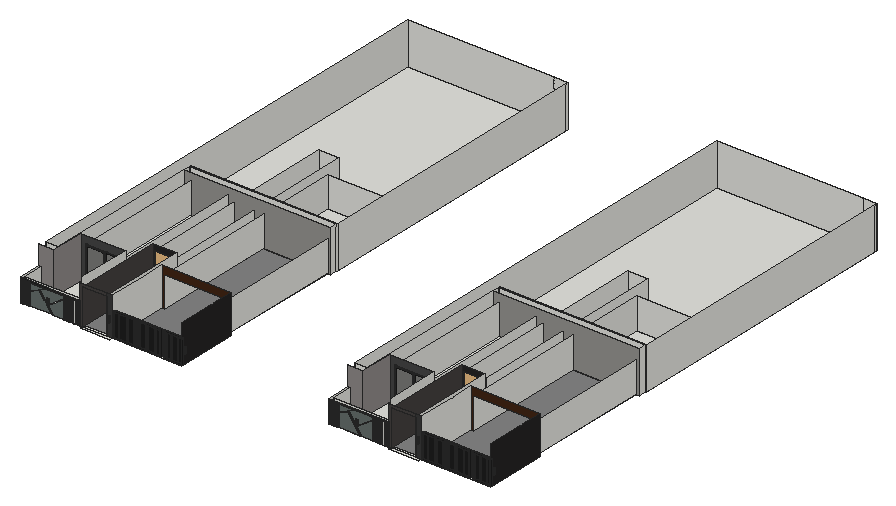
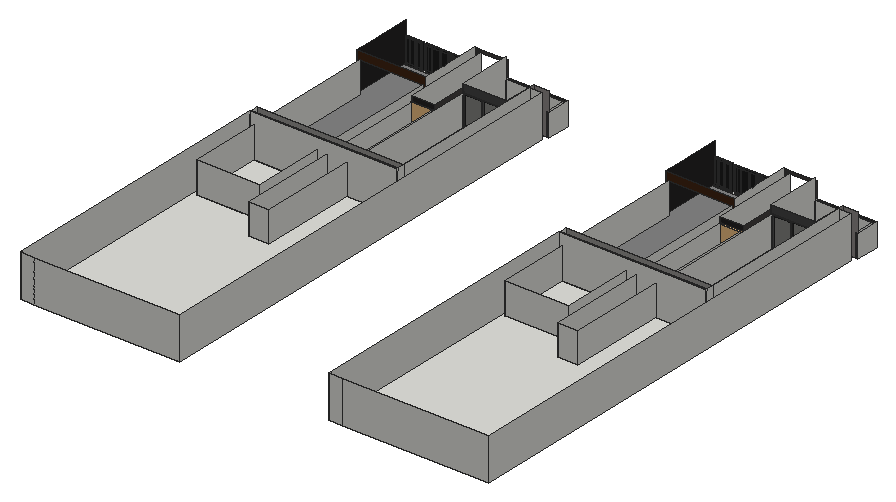
# SketchUp Ruby script. Lengths in inches.
U = 1.inch
M = Sketchup.active_model
def pt(a) = Geom::Point3d.new(a.map { |v| v * U })
def face(e, loops, mat)
  f = e.add_face(loops[0].map { |a| pt(a) })
  loops[1..].each { |l| e.add_face(l.map { |a| pt(a) }).erase! }
  f.material = f.back_material = mat if mat
  f
end
# faces: each face lists its corners as indices into pts; further lists are holes
def faces(e, pts, list, mat = nil) = list.each { |f| face(e, (f[0].is_a?(Array) ? f : [f]).map { |l| l.map { |i| pts[i] } }, mat) }
# xy, xz, yz: faces in a plane at the given z, y or x. An outline is a flat list of corners, or four numbers for a rectangle; further outlines are holes
def ring(l) = l.size == 4 ? [[l[0], l[1]], [l[2], l[1]], [l[2], l[3]], [l[0], l[3]]] : l.each_slice(2).to_a
def flat(e, list, mat, &to3) = list.each { |f| face(e, (f[0].is_a?(Array) ? f : [f]).map { |l| ring(l).map { |u, v| to3.(u, v) } }, mat) }
def xy(e, z, list, mat = nil) = flat(e, list, mat) { |x, y| [x, y, z] }
def xz(e, y, list, mat = nil) = flat(e, list, mat) { |x, z| [x, y, z] }
def yz(e, x, list, mat = nil) = flat(e, list, mat) { |y, z| [x, y, z] }
def lines(e, pts, list) = list.each { |a, b| e.add_line(pt(pts[a]), pt(pts[b])) }
# prism: a flat outline (further loops are holes) pulled along v
def prism(e, loops, v, mat = nil)
  f = face(e, loops, mat); d = Geom::Vector3d.new(v.map { |x| x * U })
  f.pushpull(f.normal.samedirection?(d) ? d.length : -d.length)
end
def box(e, o, s, mat = nil) = prism(e, [[o, [o[0] + s[0], o[1], o[2]], [o[0] + s[0], o[1] + s[1], o[2]], [o[0], o[1] + s[1], o[2]]]], [0, 0, s[2]], mat)
def at(x, y, z, deg = 0) = Geom::Transformation.translation(pt([x, y, z])) * Geom::Transformation.rotation(ORIGIN, Z_AXIS, deg.degrees)
def axes(o, x, y, z) = Geom::Transformation.new([*x, 0, *y, 0, *z, 0, *pt(o).to_a, 1])
def part(name) = M.definitions.add(name)
# library, detail: a bought-in or finely detailed component or shape, given as its bounding box
def library(name, o, s) = part(name).tap { |d| box(d.entities, o, s) }
def detail(e, o, s) = box(e.add_group.entities, o, s)
def put(e, d, t, mat = nil) = e.add_instance(d, t).tap { |i| i.material = mat if mat }
def group(e, t, mat = nil) = e.add_group.tap { |g| g.transformation = t; g.material = mat if mat }.entities
root = M.entities
M.materials.add("Glass_Tinted_Gray").color = [0, 0, 0]
M.materials["Glass_Tinted_Gray"].alpha = 0.125
M.materials.add("[0135_DarkGray]").color = [81, 81, 81]
M.materials.add("[Color M07]").color = [58, 58, 58]
M.materials.add("[Color M08]").color = [30, 30, 30]
M.materials.add("[Granite Dark Gray]").color = [38, 37, 37]
M.materials.add("[Granite Dark Gray]1").color = [69, 68, 68]
M.materials.add("[Granite Light Gray]").color = [149, 148, 144]
M.materials.add("[Granite Tile]1").color = [68, 65, 63]
M.materials.add("[Mirror 02]").color = [229, 229, 229]
M.materials.add("[Slate]").color = [102, 110, 108]
M.materials.add("[Stone Marble]").color = [143, 138, 136]
M.materials.add("[Terrazzo Light Blue]").color = [196, 214, 227]
M.materials.add("[Tile Grey]").color = [132, 132, 132]
M.materials.add("[Wood Veneer 01]").color = [66, 38, 20]
c1 = part("Group\#7")
xy(c1.entities,0,[[6,0,4.45,0.2,3,0.8,1.76,1.76,0.8,3,0.2,4.45,0,6,0.2,7.55,0.8,9,1.76,10.24,3,11.2,4.45,11.8,6,12,7.55,11.8,9,11.2,10.24,10.24,11.2,9,11.8,7.55,12,6,11.8,4.45,11.2,3,10.24,1.76,9,0.8,7.55,0.2]])
xy(c1.entities,37,[[6,0,7.55,0.2,9,0.8,10.24,1.76,11.2,3,11.8,4.45,12,6,11.8,7.55,11.2,9,10.24,10.24,9,11.2,7.55,11.8,6,12,4.45,11.8,3,11.2,1.76,10.24,0.8,9,0.2,7.55,0,6,0.2,4.45,0.8,3,1.76,1.76,3,0.8,4.45,0.2]],"[Granite Tile]1")
p = [[4.45,0.2,0],[6,0,0],[6,0,37],[4.45,0.2,37],[7.55,0.2,0],[7.55,0.2,37],
  [3,0.8,0],[3,0.8,37],[9,0.8,0],[9,0.8,37],[1.76,1.76,0],[1.76,1.76,37],
  [10.24,1.76,0],[10.24,1.76,37],[0.8,3,0],[0.8,3,37],[11.2,3,0],[11.2,3,37],
  [0.2,4.45,0],[0.2,4.45,37],[11.8,4.45,0],[11.8,4.45,37],[0,6,0],[0,6,37],
  [12,6,0],[12,6,37],[0.2,7.55,0],[0.2,7.55,37],[11.8,7.55,0],[11.8,7.55,37],
  [0.8,9,0],[0.8,9,37],[11.2,9,0],[11.2,9,37],[1.76,10.24,0],[1.76,10.24,37],
  [10.24,10.24,0],[10.24,10.24,37],[3,11.2,0],[3,11.2,37],[9,11.2,0],[9,11.2,37],
  [4.45,11.8,0],[4.45,11.8,37],[7.55,11.8,0],[7.55,11.8,37],[6,12,0],[6,12,37]]
faces(c1.entities,p,[[0,1,2,3],[1,4,5,2],[6,0,3,7],[4,8,9,5],[10,6,7,11],[8,12,13,9],[14,10,11,15],[12,16,17,13],
  [18,14,15,19],[16,20,21,17],[22,18,19,23],[20,24,25,21],[26,22,23,27],[24,28,29,25],[30,26,27,31],[28,32,33,29],
  [34,30,31,35],[32,36,37,33],[38,34,35,39],[36,40,41,37],[42,38,39,43],[40,44,45,41],[46,42,43,47],[44,46,47,45]],"[Granite Tile]1")
c2 = part("PENTEK_RP Fineline 50S_Sliding_DoorCase_E1")
box(c2.entities,[0,0,0],[1.51,3.66,99.27],"[0135_DarkGray]")
c3 = part("PENTEK_RP Fineline 50S_SlidingDooe_Case_E2")
box(c3.entities,[0,0,0],[96.25,3.66,1.51],"[0135_DarkGray]")
c4 = part("pentek_RP Fineline 50S_SlidingDoor_Case")
put(c4.entities,c2,at(97.76,0,0))
put(c4.entities,c3,at(1.51,0,0))
put(c4.entities,c2,at(0,0,0))
put(c4.entities,c3,at(1.51,0,97.76))
c5 = part("PENTEK_RP Fineline 50S_SlidingDoor_GlazingBead_2")
box(c5.entities,[0,0,0],[0.56,0.59,94.39],"[0135_DarkGray]")
c6 = part("PENTEK_RP Fineline 50S_SlidingDoor_Glass")
box(c6.entities,[0,0,0],[46.58,0.16,94.39],"Glass_Tinted_Gray")
c7 = part("PENTEK_RP Fineline 50S_SlidingDoor_GlazingBead")
box(c7.entities,[0,0,0],[45.47,0.59,0.56],"[0135_DarkGray]")
c8 = part("PENTEK_RP Fineline 50S_SlidingDoor_Leaf_E1")
xy(c8.entities,0,[[0,0,0.93,1.97],[0.93,1.57,1.49,1.97]],"[0135_DarkGray]")
xy(c8.entities,96.25,[[0,0,0.93,0,0.93,1.57,1.49,1.57,1.49,1.97,0,1.97]],"[0135_DarkGray]")
xz(c8.entities,0,[[0,0,0.93,96.25]],"[0135_DarkGray]")
xz(c8.entities,1.57,[[0.93,0,1.49,95.32],[0.93,95.32,1.49,96.25]],"[0135_DarkGray]")
xz(c8.entities,1.97,[[0,0,1.49,96.25]],"[0135_DarkGray]")
yz(c8.entities,0,[[0,0,1.97,96.25]],"[0135_DarkGray]")
yz(c8.entities,0.93,[[0,0,1.57,0.93],[0,0.93,1.57,95.32],[0,95.32,1.57,96.25]],"[0135_DarkGray]")
yz(c8.entities,1.49,[[1.57,0,1.97,95.32],[1.57,95.32,1.97,96.25]],"[0135_DarkGray]")
c9 = part("PENTEK_RP Fineline 50S_SlidingDoor_Leaf_E2")
xy(c9.entities,0,[[0,0,0,1.57,0.56,1.57,0.56,1.97,46.02,1.97,46.02,1.57,46.58,1.57,46.58,0]],"[0135_DarkGray]")
xy(c9.entities,0.93,[[0,0,46.58,1.57]],"[0135_DarkGray]")
xy(c9.entities,1.49,[[0.56,1.57,46.02,1.97]],"[0135_DarkGray]")
xz(c9.entities,0,[[0,0,46.58,0.93]],"[0135_DarkGray]")
xz(c9.entities,1.57,[[0,0,0.56,0.93],[46.02,0,46.58,0.93],[0.56,0.93,46.02,1.49]],"[0135_DarkGray]")
xz(c9.entities,1.97,[[0.56,0,46.02,1.49]],"[0135_DarkGray]")
yz(c9.entities,0,[[0,0,1.57,0.93]],"[0135_DarkGray]")
yz(c9.entities,0.56,[[1.57,0,1.97,0.93],[1.57,0.93,1.97,1.49]],"[0135_DarkGray]")
yz(c9.entities,46.02,[[1.57,0,1.97,0.93],[1.57,0.93,1.97,1.49]],"[0135_DarkGray]")
yz(c9.entities,46.58,[[0,0,1.57,0.93]],"[0135_DarkGray]")
c10 = part("PENTEK_RP Fineline S_SlidingDoor_Leaf1")
put(c10.entities,c5,at(0.93,0,0.93))
put(c10.entities,c5,at(46.96,0,0.93))
put(c10.entities,c6,at(1.49,1.42,0.93))
put(c10.entities,c7,at(1.49,0,0.93))
put(c10.entities,c6,at(1.49,0.59,0.93),"[Terrazzo Light Blue]")
put(c10.entities,c8,at(0,0,0))
put(c10.entities,c8,axes([48.44,0,0],[-1,0,0],[0,1,0],[0,0,1]))
put(c10.entities,c9,axes([0.93,0,96.25],[1,0,0],[0,1,0],[0,0,-1]))
put(c10.entities,c9,at(0.93,0,0))
put(c10.entities,c7,at(1.49,0,94.77))
c11 = part("PENTEK_RP Fineline 50S_SlidingDoor_Leaf2")
put(c11.entities,c6,at(1.49,1.42,0.93))
put(c11.entities,c7,at(1.49,0,94.77))
put(c11.entities,c5,at(46.96,0,0.93))
put(c11.entities,c6,at(1.49,0.59,0.93),"[Mirror 02]")
put(c11.entities,c5,at(0.93,0,0.93))
put(c11.entities,c8,at(0,0,0))
put(c11.entities,c8,axes([48.44,0,0],[-1,0,0],[0,1,0],[0,0,1]))
put(c11.entities,c7,at(1.49,0,0.93))
put(c11.entities,c9,axes([0.93,0,96.25],[1,0,0],[0,1,0],[0,0,-1]))
put(c11.entities,c9,at(0.93,0,0))
c12 = part("PENTEK - Slimmest Steel Sliding Door / Window\#1")
put(c12.entities,c4,at(0,-1.88,-0.09))
put(c12.entities,c10,at(1.51,-2.27,1.42))
put(c12.entities,c11,at(49.32,-0.3,1.42))
c13 = library("元件\#5",[-4.39,0,0],[5.37,35.83,90.55])
c14 = part("Group\#102")
g1 = group(c14.entities,at(0,0,0))
prism(g1,[[[0,3,72],[70.5,3,72],[70.5,3,0],[0,3,0]],[[67.5,3,3],[67.5,3,69],[3,3,69],[3,3,3]]],[0,-3,0])
c15 = part("Group\#135")
box(c15.entities,[0,0,0],[0.5,1,66])
c16 = part("Group\#148")
box(c16.entities,[0,-1,0],[5.5,1,66])
box(c16.entities,[50.84,-1,0],[13.66,1,66])
box(c16.entities,[28.06,-1,0],[22.28,1,66])
box(c16.entities,[24.66,-1,0],[2.9,1,66])
box(c16.entities,[6,-1,0],[18.16,1,66])
c17 = part("Component\#23")
g2 = group(c17.entities,at(70.5,0,0),"[Color M08]")
put(g2,c14,axes([70.5,0,0],[-1,0,0],[0,1,0],[0,0,1]))
g3 = group(g2,at(3,2,3))
g4 = group(g3,at(0,-1,0))
box(g4,[0,0,0],[5.5,1,66])
box(g4,[50.84,0,0],[13.66,1,66])
box(g4,[28.06,0,0],[22.28,1,66])
box(g4,[24.66,0,0],[2.9,1,66])
box(g4,[6,0,0],[18.16,1,66])
put(g3,c15,axes([50.34,0,0],[1,0,0],[0,-1,0],[0,0,1]))
put(g3,c15,axes([24.16,0,0],[1,0,0],[0,-1,0],[0,0,1]))
put(g3,c15,axes([27.56,0,0],[1,0,0],[0,-1,0],[0,0,1]))
put(g3,c15,axes([5.5,0,0],[1,0,0],[0,-1,0],[0,0,1]))
g5 = group(c17.entities,at(70.5,0,0),"[Color M08]")
put(g5,c14,at(-70.5,0,0))
g6 = group(g5,at(-3,2,3,-180))
put(g6,c16,at(0,1,0))
put(g6,c15,at(50.34,0,0))
put(g6,c15,at(24.16,0,0))
put(g6,c15,at(27.56,0,0))
put(g6,c15,at(5.5,0,0))
g7 = group(c17.entities,at(150,0,0),"[Color M08]")
put(g7,c14,axes([54,0,0],[-0.76596,0,0],[0,1,0],[0,0,1]))
g8 = group(g7,at(2.3,2,3))
put(g8,c16,axes([0,-1,0],[0.76596,0,0],[0,-1,0],[0,0,1]))
put(g8,c15,axes([38.55,0,0],[0.76596,0,0],[0,-1,0],[0,0,1]))
put(g8,c15,axes([18.5,0,0],[0.76596,0,0],[0,-1,0],[0,0,1]))
put(g8,c15,axes([21.11,0,0],[0.76596,0,0],[0,-1,0],[0,0,1]))
put(g8,c15,axes([4.22,0,0],[0.76596,0,0],[0,-1,0],[0,0,1]))
xy(root,8.5,[[2153.45,2285.625,2237.65,2294.125],[3032.2,2285.625,3116.4,2294.125],[1976.47,2293.1875,1980.03,2294.125],[1981.28,2293.1875,1984.84,2294.125],[1986.1,2293.1875,1989.66,2294.125],
  [1990.91,2293.1875,1994.47,2294.125],[1995.72,2293.1875,1999.28,2294.125],[2000.53,2293.1875,2004.09,2294.125],[2100.97,2293.1875,2104.93,2294.125],[2105.97,2293.1875,2109.93,2294.125],
  [2110.97,2293.1875,2114.93,2294.125],[2115.97,2293.1875,2119.93,2294.125],[2120.97,2293.1875,2124.93,2294.125],[2125.97,2293.1875,2129.93,2294.125],[2135.7,2293.1875,2139.36,2294.125],
  [2143.16,2293.1875,2146.28,2294.125],[2855.22,2293.1875,2858.78,2294.125],[2860.03,2293.1875,2863.59,2294.125],[2864.85,2293.1875,2868.41,2294.125],[2869.66,2293.1875,2873.22,2294.125],
  [2874.47,2293.1875,2878.03,2294.125],[2879.28,2293.1875,2882.84,2294.125],[2979.72,2293.1875,2983.68,2294.125],[2984.72,2293.1875,2988.68,2294.125],[2989.72,2293.1875,2993.68,2294.125],
  [2994.72,2293.1875,2998.68,2294.125],[2999.72,2293.1875,3003.68,2294.125],[3004.72,2293.1875,3008.68,2294.125],[3014.45,2293.1875,3018.11,2294.125],[3021.91,2293.1875,3025.03,2294.125],
  [1976.47,2294.125,1976.47,2358.81,1983.29,2358.81,1983.29,2300.94,2146.28,2300.94,2146.28,2294.125,2067.62,2294.125,2067.62,2297,2064.07,2297,2064.07,2294.125],[2064.07,2294.125,2067.62,2297],[2153.45,2294.125,2221.2,2300.94],[2238.79,2294.125,2436.4,2300.94],[2855.22,2294.125,2855.22,2358.81,2862.04,2358.81,2862.04,2300.94,3025.03,2300.94,3025.03,2294.125,2946.37,2294.125,2946.37,2297,2942.82,2297,2942.82,2294.125],
  [2942.82,2294.125,2946.37,2297],[3032.2,2294.125,3099.95,2300.94],[3117.54,2294.125,3315.15,2300.94],[1983.29,2300.94,2146.28,2300.94,2146.28,2454.68,2020.16,2454.68,2020.16,2358.81,1983.29,2358.81],[2862.04,2300.94,3025.03,2300.94,3025.03,2454.68,2898.91,2454.68,2898.91,2358.81,2862.04,2358.81],
  [1983.29,2374.65,2019.03,2374.65,2019.03,2846.52,2160.47,2846.52,2160.47,3124.06,2218.35,3124.06,2218.35,2846.52,2246.4,2846.52,2246.4,3049.31,2427.3,3049.31,2427.3,2846.52,2436.4,2846.52,2436.4,3664.43,1983.29,3664.43],[2862.04,2374.65,2897.78,2374.65,2897.78,2846.52,3039.22,2846.52,3039.22,3124.06,3097.1,3124.06,3097.1,2846.52,3125.15,2846.52,3125.15,3049.31,3306.05,3049.31,3306.05,2846.52,3315.15,2846.52,3315.15,3664.43,2862.04,3664.43],[2019.03,2822.08,2160.47,2841.77],[2160.47,2822.08,2218.35,2841.77],[2218.35,2822.08,2246.4,2841.77],
  [2246.4,2822.08,2427.3,2841.77],[2427.3,2822.08,2436.4,2841.77],[2897.78,2822.08,3039.22,2841.77],[3039.22,2822.08,3097.1,2841.77],[3097.1,2822.08,3125.15,2841.77],
  [3125.15,2822.08,3306.05,2841.77],[3306.05,2822.08,3315.15,2841.77],[2019.03,2841.77,2160.47,2846.52],[2160.47,2841.77,2218.35,2846.52],[2218.35,2841.77,2246.4,2846.52],
  [2246.4,2841.77,2427.3,2846.52],[2427.3,2841.77,2436.4,2846.52],[2897.78,2841.77,3039.22,2846.52],[3039.22,2841.77,3097.1,2846.52],[3097.1,2841.77,3125.15,2846.52],
  [3125.15,2841.77,3306.05,2846.52],[3306.05,2841.77,3315.15,2846.52],[2160.47,2846.52,2218.35,3124.06],[2246.4,2846.52,2427.3,3049.31],[3039.22,2846.52,3097.1,3124.06],
  [3125.15,2846.52,3306.05,3049.31]])
xy(root,8.5,[[2153.45,2300.94,2221.2,2300.94,2221.2,2542.24,2218.35,2542.24,2218.35,2822.08,2160.47,2822.08,2160.47,2542.24,2153.45,2542.24],[2238.79,2300.94,2436.4,2300.94,2436.4,2468.68,2427.3,2468.68,2427.3,2822.08,2246.4,2822.08,2246.4,2468.68,2238.79,2468.68],[3032.2,2300.94,3099.95,2300.94,3099.95,2542.24,3097.1,2542.24,3097.1,2822.08,3039.22,2822.08,3039.22,2542.24,3032.2,2542.24],[3117.54,2300.94,3315.15,2300.94,3315.15,2468.68,3306.05,2468.68,3306.05,2822.08,3125.15,2822.08,3125.15,2468.68,3117.54,2468.68]],"[Tile Grey]")
xy(root,20.01,[[2037.38,2454.68,2142.51,2841.77],[2916.13,2454.68,3021.26,2841.77]])
xy(root,68.78,[[1980.03,2293.1875,1981.28,2294.125],[1984.84,2293.1875,1986.1,2294.125],[1989.66,2293.1875,1990.91,2294.125],[1994.47,2293.1875,1995.72,2294.125],[1999.28,2293.1875,2000.53,2294.125],
  [2004.09,2293.1875,2004.09,2294.125,2047.85,2294.125,2047.85,2297,2050.98,2297,2050.98,2294.125,2100.97,2294.125,2100.97,2293.1875],[2104.93,2293.1875,2105.97,2294.125],[2109.93,2293.1875,2110.97,2294.125],[2114.93,2293.1875,2115.97,2294.125],[2119.93,2293.1875,2120.97,2294.125],
  [2124.93,2293.1875,2125.97,2294.125],[2129.93,2293.1875,2135.7,2294.125],[2139.36,2293.1875,2143.16,2294.125],[2858.78,2293.1875,2860.03,2294.125],[2863.59,2293.1875,2864.85,2294.125],
  [2868.41,2293.1875,2869.66,2294.125],[2873.22,2293.1875,2874.47,2294.125],[2878.03,2293.1875,2879.28,2294.125],[2882.84,2293.1875,2882.84,2294.125,2926.6,2294.125,2926.6,2297,2929.73,2297,2929.73,2294.125,2979.72,2294.125,2979.72,2293.1875],[2983.68,2293.1875,2984.72,2294.125],
  [2988.68,2293.1875,2989.72,2294.125],[2993.68,2293.1875,2994.72,2294.125],[2998.68,2293.1875,2999.72,2294.125],[3003.68,2293.1875,3004.72,2294.125],[3008.68,2293.1875,3014.45,2294.125],
  [3018.11,2293.1875,3021.91,2294.125]])
xz(root,2293.1875,[[1976.47,8.5,1980.03,68.78],[1981.28,8.5,1984.84,68.78],[1986.1,8.5,1989.66,68.78],[1990.91,8.5,1994.47,68.78],[1995.72,8.5,1999.28,68.78],
  [2000.53,8.5,2004.09,68.78],[2100.97,8.5,2104.93,68.78],[2105.97,8.5,2109.93,68.78],[2110.97,8.5,2114.93,68.78],[2115.97,8.5,2119.93,68.78],
  [2120.97,8.5,2124.93,68.78],[2143.16,8.5,2146.28,68.78],[2855.22,8.5,2858.78,68.78],[2860.03,8.5,2863.59,68.78],[2864.85,8.5,2868.41,68.78],
  [2869.66,8.5,2873.22,68.78],[2874.47,8.5,2878.03,68.78],[2879.28,8.5,2882.84,68.78],[2979.72,8.5,2983.68,68.78],[2984.72,8.5,2988.68,68.78],
  [2989.72,8.5,2993.68,68.78],[2994.72,8.5,2998.68,68.78],[2999.72,8.5,3003.68,68.78],[3021.91,8.5,3025.03,68.78],[1976.47,68.78,2146.28,72.4375],
  [2855.22,68.78,3025.03,72.4375]],"[Color M08]")
xz(root,2293.1875,[[2125.97,8.5,2129.93,68.78],[2135.7,8.5,2139.36,68.78],[3004.72,8.5,3008.68,68.78],[3014.45,8.5,3018.11,68.78]],"[Slate]")
xz(root,2294.125,[[1980.03,8.5,1981.28,68.78],[1984.84,8.5,1986.1,68.78],[1989.66,8.5,1990.91,68.78],[1994.47,8.5,1995.72,68.78],[1999.28,8.5,2000.53,68.78],
  [2104.93,8.5,2105.97,68.78],[2109.93,8.5,2110.97,68.78],[2114.93,8.5,2115.97,68.78],[2119.93,8.5,2120.97,68.78],[2124.93,8.5,2125.97,68.78],
  [2858.78,8.5,2860.03,68.78],[2863.59,8.5,2864.85,68.78],[2868.41,8.5,2869.66,68.78],[2873.22,8.5,2874.47,68.78],[2878.03,8.5,2879.28,68.78],
  [2983.68,8.5,2984.72,68.78],[2988.68,8.5,2989.72,68.78],[2993.68,8.5,2994.72,68.78],[2998.68,8.5,2999.72,68.78],[3003.68,8.5,3004.72,68.78]])
xz(root,2294.125,[[2221.2,8.5,2238.79,118.38],[3099.95,8.5,3117.54,118.38]],"[Color M07]")
xz(root,2294.125,[[2129.93,8.5,2135.7,68.78],[2139.36,8.5,2143.16,68.78],[3008.68,8.5,3014.45,68.78],[3018.11,8.5,3021.91,68.78]],"[Color M08]")
xz(root,2294.125,[[2146.28,8.5,2153.45,8.5,2153.45,110.32,2221.2,110.32,2221.2,118.38,2146.28,118.38],[3025.03,8.5,3032.2,8.5,3032.2,110.32,3099.95,110.32,3099.95,118.38,3025.03,118.38]],"[Granite Tile]1")
xz(root,2294.125,[[2004.09,8.5,2064.07,8.5,2029.37,57.375,2004.09,44.04],[2067.62,8.5,2100.97,8.5,2100.97,58.8,2055.31,25.91],[2882.84,8.5,2942.82,8.5,2908.12,57.375,2882.84,44.04],[2946.37,8.5,2979.72,8.5,2979.72,58.8,2934.06,25.91],[2052.89,29.34,2100.97,62.06,2100.97,68.78,2050.98,68.78,2032.07,58.8],
  [2931.64,29.34,2979.72,62.06,2979.72,68.78,2929.73,68.78,2910.82,58.8],[2004.09,46.32,2047.85,68.78,2004.09,68.78],[2882.84,46.32,2926.6,68.78,2882.84,68.78]],"[Slate]")
xz(root,2297,[[2064.07,8.5,2067.62,8.5,2055.31,25.91,2052.89,29.34,2032.07,58.8,2029.37,57.375],[2942.82,8.5,2946.37,8.5,2934.06,25.91,2931.64,29.34,2910.82,58.8,2908.12,57.375],[2055.31,25.91,2100.97,58.8,2100.97,62.06,2052.89,29.34],[2934.06,25.91,2979.72,58.8,2979.72,62.06,2931.64,29.34],[2004.09,44.04,2029.37,57.375,2032.07,58.8,2050.98,68.78,2047.85,68.78,2004.09,46.32],
  [2882.84,44.04,2908.12,57.375,2910.82,58.8,2929.73,68.78,2926.6,68.78,2882.84,46.32]])
xz(root,2300.94,[[1983.29,8.5,2146.28,72.4375],[2862.04,8.5,3025.03,72.4375]])
xz(root,2358.81,[[1976.47,8.5,1983.29,72.4375],[2855.22,8.5,2862.04,72.4375]])
xz(root,2358.81,[[1983.29,8.5,2020.16,8.5,2020.16,128.5,1976.47,128.5,1976.47,72.4375,1983.29,72.4375],[2862.04,8.5,2898.91,8.5,2898.91,128.5,2855.22,128.5,2855.22,72.4375,2862.04,72.4375]],"[Stone Marble]")
xz(root,2374.65,[[1983.29,8.5,2019.03,128.5],[2862.04,8.5,2897.78,128.5]])
xz(root,2454.68,[[[2020.16,8.5,2146.28,128.5],[2037.38,20.01,2142.51,107.07]],[[2898.91,8.5,3025.03,128.5],[2916.13,20.01,3021.26,107.07]]],"[Granite Dark Gray]1")
xz(root,2468.68,[[2238.79,8.5,2246.4,8.5,2246.4,96.29,2427.3,96.29,2427.3,8.5,2436.4,8.5,2436.4,118.38,2238.79,118.38],[3117.54,8.5,3125.15,8.5,3125.15,96.29,3306.05,96.29,3306.05,8.5,3315.15,8.5,3315.15,118.38,3117.54,118.38]],"[Wood Veneer 01]")
xz(root,2542.24,[[2153.45,8.5,2160.47,8.5,2160.47,96.1875,2218.35,96.1875,2218.35,8.5,2221.2,8.5,2221.2,110.32,2153.45,110.32],[3032.2,8.5,3039.22,8.5,3039.22,96.1875,3097.1,96.1875,3097.1,8.5,3099.95,8.5,3099.95,110.32,3032.2,110.32]],"[Granite Dark Gray]")
xz(root,2822.08,[[2019.03,8.5,2436.4,128.5],[2897.78,8.5,3315.15,128.5]],"[Granite Light Gray]")
xz(root,2841.77,[[[2019.03,8.5,2436.4,128.5],[2037.38,20.01,2142.51,107.07]],[[2897.78,8.5,3315.15,128.5],[2916.13,20.01,3021.26,107.07]]])
xz(root,2846.52,[[2019.03,8.5,2436.4,128.5],[2897.78,8.5,3315.15,128.5]])
xz(root,3049.31,[[2246.4,8.5,2427.3,96.29],[3125.15,8.5,3306.05,96.29]])
xz(root,3124.06,[[2160.47,8.5,2218.35,96.1875],[3039.22,8.5,3097.1,96.1875]])
xz(root,3664.43,[[1983.29,8.5,2397.9,128.5],[2397.9,8.5,2436.4,128.5],[2862.04,8.5,3276.65,128.5],[3276.65,8.5,3315.15,128.5]])
yz(root,1976.47,[[2293.1875,8.5,2358.81,72.4375]])
yz(root,1980.03,[[2293.1875,8.5,2294.125,68.78]])
yz(root,1981.28,[[2293.1875,8.5,2294.125,68.78]])
yz(root,1983.29,[[2300.94,8.5,2358.81,72.4375],[2374.65,8.5,3664.43,128.5]])
yz(root,1984.84,[[2293.1875,8.5,2294.125,68.78]])
yz(root,1986.1,[[2293.1875,8.5,2294.125,68.78]])
yz(root,1989.66,[[2293.1875,8.5,2294.125,68.78]])
yz(root,1990.91,[[2293.1875,8.5,2294.125,68.78]])
yz(root,1994.47,[[2293.1875,8.5,2294.125,68.78]])
yz(root,1995.72,[[2293.1875,8.5,2294.125,68.78]])
yz(root,1999.28,[[2293.1875,8.5,2294.125,68.78]])
yz(root,2000.53,[[2293.1875,8.5,2294.125,68.78]])
yz(root,2004.09,[[2293.1875,8.5,2294.125,8.5,2294.125,44.04,2297,44.04,2297,46.32,2294.125,46.32,2294.125,68.78,2293.1875,68.78]])
yz(root,2019.03,[[2374.65,8.5,2822.08,128.5],[2822.08,8.5,2841.77,128.5],[2841.77,8.5,2846.52,128.5]])
yz(root,2020.16,[[2358.81,8.5,2454.68,128.5]],"[Stone Marble]")
yz(root,2037.38,[[2454.68,20.01,2841.77,107.07]])
yz(root,2100.97,[[2293.1875,8.5,2293.1875,68.78,2294.125,68.78,2294.125,62.06,2297,62.06,2297,58.8,2294.125,58.8,2294.125,8.5]])
yz(root,2104.93,[[2293.1875,8.5,2294.125,68.78]])
yz(root,2105.97,[[2293.1875,8.5,2294.125,68.78]])
yz(root,2109.93,[[2293.1875,8.5,2294.125,68.78]])
yz(root,2110.97,[[2293.1875,8.5,2294.125,68.78]])
yz(root,2114.93,[[2293.1875,8.5,2294.125,68.78]])
yz(root,2115.97,[[2293.1875,8.5,2294.125,68.78]])
yz(root,2119.93,[[2293.1875,8.5,2294.125,68.78]])
yz(root,2120.97,[[2293.1875,8.5,2294.125,68.78]])
yz(root,2124.93,[[2293.1875,8.5,2294.125,68.78]])
yz(root,2125.97,[[2293.1875,8.5,2294.125,68.78]])
yz(root,2129.93,[[2293.1875,8.5,2294.125,68.78]])
yz(root,2135.7,[[2293.1875,8.5,2294.125,68.78]])
yz(root,2139.36,[[2293.1875,8.5,2294.125,68.78]])
yz(root,2142.51,[[2454.68,20.01,2841.77,107.07]])
yz(root,2143.16,[[2293.1875,8.5,2294.125,68.78]])
yz(root,2146.28,[[2293.1875,8.5,2294.125,68.78],[2294.125,8.5,2300.94,72.4375],[2300.94,8.5,2454.68,128.5],[2293.1875,68.78,2294.125,72.4375]])
yz(root,2153.45,[[2294.125,8.5,2542.24,110.32]],"[Granite Tile]1")
yz(root,2160.47,[[2542.24,8.5,3124.06,96.1875]])
yz(root,2218.35,[[2542.24,8.5,3124.06,96.1875]])
yz(root,2221.2,[[2294.125,8.5,2542.24,110.32]])
yz(root,2238.79,[[2294.125,8.5,2468.68,8.5,2468.68,118.38,2407.27,118.38,2407.27,116.94,2396.68,116.94,2396.68,118.38,2294.125,118.38]])
yz(root,2246.4,[[2468.68,8.5,3049.31,96.29]])
yz(root,2427.3,[[2468.68,8.5,3049.31,96.29]])
yz(root,2436.4,[[2822.08,8.5,2841.77,128.5],[2841.77,8.5,2846.52,128.5],[2846.52,8.5,3658.44,128.5],[3658.44,8.5,3664.43,128.5]])
yz(root,2436.4,[[2294.125,8.5,2294.125,118.38,2396.68,118.38,2396.68,116.94,2407.27,116.94,2407.27,118.38,2468.68,118.38,2468.68,8.5]],"[Granite Dark Gray]")
yz(root,2855.22,[[2293.1875,8.5,2358.81,72.4375]])
yz(root,2858.78,[[2293.1875,8.5,2294.125,68.78]])
yz(root,2860.03,[[2293.1875,8.5,2294.125,68.78]])
yz(root,2862.04,[[2300.94,8.5,2358.81,72.4375],[2374.65,8.5,3664.43,128.5]])
yz(root,2863.59,[[2293.1875,8.5,2294.125,68.78]])
yz(root,2864.85,[[2293.1875,8.5,2294.125,68.78]])
yz(root,2868.41,[[2293.1875,8.5,2294.125,68.78]])
yz(root,2869.66,[[2293.1875,8.5,2294.125,68.78]])
yz(root,2873.22,[[2293.1875,8.5,2294.125,68.78]])
yz(root,2874.47,[[2293.1875,8.5,2294.125,68.78]])
yz(root,2878.03,[[2293.1875,8.5,2294.125,68.78]])
yz(root,2879.28,[[2293.1875,8.5,2294.125,68.78]])
yz(root,2882.84,[[2293.1875,8.5,2294.125,8.5,2294.125,44.04,2297,44.04,2297,46.32,2294.125,46.32,2294.125,68.78,2293.1875,68.78]])
yz(root,2897.78,[[2374.65,8.5,2822.08,128.5],[2822.08,8.5,2841.77,128.5],[2841.77,8.5,2846.52,128.5]])
yz(root,2898.91,[[2358.81,8.5,2454.68,128.5]],"[Stone Marble]")
yz(root,2916.13,[[2454.68,20.01,2841.77,107.07]])
yz(root,2979.72,[[2293.1875,8.5,2293.1875,68.78,2294.125,68.78,2294.125,62.06,2297,62.06,2297,58.8,2294.125,58.8,2294.125,8.5]])
yz(root,2983.68,[[2293.1875,8.5,2294.125,68.78]])
yz(root,2984.72,[[2293.1875,8.5,2294.125,68.78]])
yz(root,2988.68,[[2293.1875,8.5,2294.125,68.78]])
yz(root,2989.72,[[2293.1875,8.5,2294.125,68.78]])
yz(root,2993.68,[[2293.1875,8.5,2294.125,68.78]])
yz(root,2994.72,[[2293.1875,8.5,2294.125,68.78]])
yz(root,2998.68,[[2293.1875,8.5,2294.125,68.78]])
yz(root,2999.72,[[2293.1875,8.5,2294.125,68.78]])
yz(root,3003.68,[[2293.1875,8.5,2294.125,68.78]])
yz(root,3004.72,[[2293.1875,8.5,2294.125,68.78]])
yz(root,3008.68,[[2293.1875,8.5,2294.125,68.78]])
yz(root,3014.45,[[2293.1875,8.5,2294.125,68.78]])
yz(root,3018.11,[[2293.1875,8.5,2294.125,68.78]])
yz(root,3021.26,[[2454.68,20.01,2841.77,107.07]])
yz(root,3021.91,[[2293.1875,8.5,2294.125,68.78]])
yz(root,3025.03,[[2293.1875,8.5,2294.125,68.78],[2294.125,8.5,2300.94,72.4375],[2300.94,8.5,2454.68,128.5],[2293.1875,68.78,2294.125,72.4375]])
yz(root,3032.2,[[2294.125,8.5,2542.24,110.32]],"[Granite Tile]1")
yz(root,3039.22,[[2542.24,8.5,3124.06,96.1875]])
yz(root,3097.1,[[2542.24,8.5,3124.06,96.1875]])
yz(root,3099.95,[[2294.125,8.5,2542.24,110.32]])
yz(root,3117.54,[[2294.125,8.5,2468.68,8.5,2468.68,118.38,2407.27,118.38,2407.27,116.94,2396.68,116.94,2396.68,118.38,2294.125,118.38]])
yz(root,3125.15,[[2468.68,8.5,3049.31,96.29]])
yz(root,3306.05,[[2468.68,8.5,3049.31,96.29]])
yz(root,3315.15,[[2822.08,8.5,2841.77,128.5],[2841.77,8.5,2846.52,128.5],[2846.52,8.5,3658.44,128.5],[3658.44,8.5,3664.43,128.5]])
yz(root,3315.15,[[2294.125,8.5,2294.125,118.38,2396.68,118.38,2396.68,116.94,2407.27,116.94,2407.27,118.38,2468.68,118.38,2468.68,8.5]],"[Granite Dark Gray]")
p = [[2029.37,2294.125,57.375],[2064.07,2294.125,8.5],[2064.07,2297,8.5],[2029.37,2297,57.375],[2067.62,2294.125,8.5],[2055.31,2294.125,25.91],
  [2055.31,2297,25.91],[2067.62,2297,8.5],[2908.12,2294.125,57.375],[2942.82,2294.125,8.5],[2942.82,2297,8.5],[2908.12,2297,57.375],
  [2946.37,2294.125,8.5],[2934.06,2294.125,25.91],[2934.06,2297,25.91],[2946.37,2297,8.5],[2100.97,2294.125,58.8],[2100.97,2297,58.8],
  [2979.72,2294.125,58.8],[2979.72,2297,58.8],[2052.89,2294.125,29.34],[2032.07,2294.125,58.8],[2032.07,2297,58.8],[2052.89,2297,29.34],
  [2100.97,2294.125,62.06],[2100.97,2297,62.06],[2931.64,2294.125,29.34],[2910.82,2294.125,58.8],[2910.82,2297,58.8],[2931.64,2297,29.34],
  [2979.72,2294.125,62.06],[2979.72,2297,62.06],[2004.09,2294.125,44.04],[2004.09,2297,44.04],[2882.84,2294.125,44.04],[2882.84,2297,44.04],
  [2047.85,2294.125,68.78],[2004.09,2294.125,46.32],[2004.09,2297,46.32],[2047.85,2297,68.78],[2926.6,2294.125,68.78],[2882.84,2294.125,46.32],
  [2882.84,2297,46.32],[2926.6,2297,68.78],[2050.98,2294.125,68.78],[2050.98,2297,68.78],[2929.73,2294.125,68.78],[2929.73,2297,68.78]]
faces(root,p,[[0,1,2,3],[4,5,6,7],[8,9,10,11],[12,13,14,15],[5,16,17,6],[13,18,19,14],[20,21,22,23],[24,20,23,25],
  [26,27,28,29],[30,26,29,31],[32,0,3,33],[34,8,11,35],[36,37,38,39],[40,41,42,43],[21,44,45,22],[27,46,47,28]])
put(root,c1,axes([2051.85,2291.96,29.51],[0.42,0,0],[0,0.42,0],[0,0,0.42]))
put(root,c12,axes([2034.38,2454.68,20],[1.08916,0,0],[0,1,0],[0,0,0.87793]))
put(root,c13,axes([2160.47,2542.62,8.5],[0,-1,0],[1.61541,0,0],[0,0,0.96838]))
put(root,c1,axes([2227.28,2289.08,47.16],[0.42,0,0],[0,0.42,0],[0,0,0.42]))
put(root,c17,axes([2238.79,2294.125,8.5],[0.9687,0,0],[0,1,0],[0,0,1]))
put(root,c1,axes([2443.36,2289.09,44.5],[0.42,0,0],[0,0.42,0],[0,0,0.42]))
put(root,c1,axes([2930.6,2291.96,29.51],[0.42,0,0],[0,0.42,0],[0,0,0.42]))
put(root,c12,axes([2913.13,2454.68,20],[1.08916,0,0],[0,1,0],[0,0,0.87793]))
put(root,c13,axes([3039.22,2542.62,8.5],[0,-1,0],[1.61541,0,0],[0,0,0.96838]))
put(root,c1,axes([3106.03,2289.08,47.16],[0.42,0,0],[0,0.42,0],[0,0,0.42]))
put(root,c17,axes([3117.54,2294.125,8.5],[0.9687,0,0],[0,1,0],[0,0,1]))
put(root,c1,axes([3322.11,2289.09,44.5],[0.42,0,0],[0,0.42,0],[0,0,0.42]))
